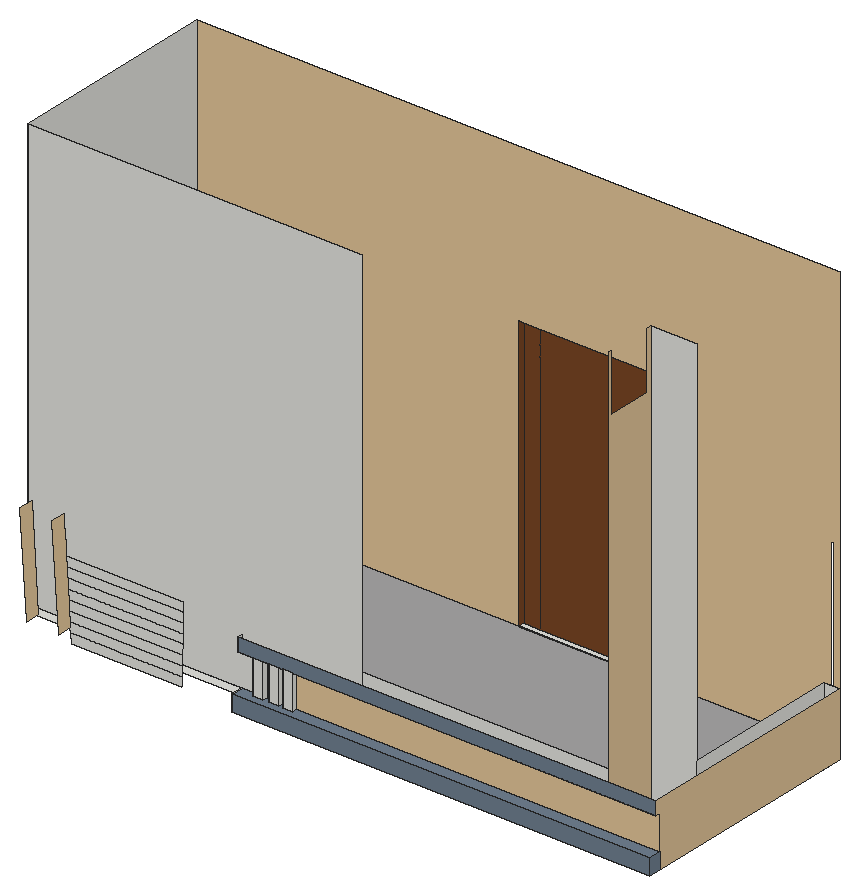
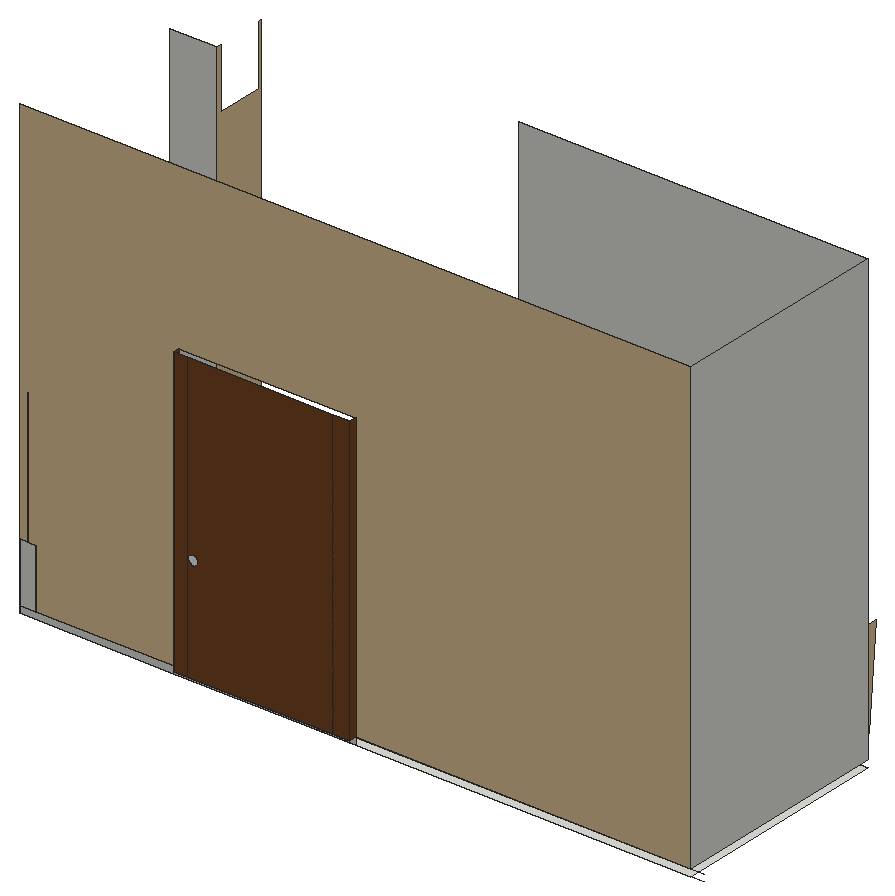
# SketchUp Ruby script. Lengths in inches.
U = 1.inch
M = Sketchup.active_model
def pt(a) = Geom::Point3d.new(a.map { |v| v * U })
def face(e, loops, mat)
  f = e.add_face(loops[0].map { |a| pt(a) })
  loops[1..].each { |l| e.add_face(l.map { |a| pt(a) }).erase! }
  f.material = f.back_material = mat if mat
  f
end
# faces: each face lists its corners as indices into pts; further lists are holes
def faces(e, pts, list, mat = nil) = list.each { |f| face(e, (f[0].is_a?(Array) ? f : [f]).map { |l| l.map { |i| pts[i] } }, mat) }
# xy, xz, yz: faces in a plane at the given z, y or x. An outline is a flat list of corners, or four numbers for a rectangle; further outlines are holes
def ring(l) = l.size == 4 ? [[l[0], l[1]], [l[2], l[1]], [l[2], l[3]], [l[0], l[3]]] : l.each_slice(2).to_a
def flat(e, list, mat, &to3) = list.each { |f| face(e, (f[0].is_a?(Array) ? f : [f]).map { |l| ring(l).map { |u, v| to3.(u, v) } }, mat) }
def xy(e, z, list, mat = nil) = flat(e, list, mat) { |x, y| [x, y, z] }
def xz(e, y, list, mat = nil) = flat(e, list, mat) { |x, z| [x, y, z] }
def yz(e, x, list, mat = nil) = flat(e, list, mat) { |y, z| [x, y, z] }
def lines(e, pts, list) = list.each { |a, b| e.add_line(pt(pts[a]), pt(pts[b])) }
# prism: a flat outline (further loops are holes) pulled along v
def prism(e, loops, v, mat = nil)
  f = face(e, loops, mat); d = Geom::Vector3d.new(v.map { |x| x * U })
  f.pushpull(f.normal.samedirection?(d) ? d.length : -d.length)
end
def box(e, o, s, mat = nil) = prism(e, [[o, [o[0] + s[0], o[1], o[2]], [o[0] + s[0], o[1] + s[1], o[2]], [o[0], o[1] + s[1], o[2]]]], [0, 0, s[2]], mat)
def at(x, y, z, deg = 0) = Geom::Transformation.translation(pt([x, y, z])) * Geom::Transformation.rotation(ORIGIN, Z_AXIS, deg.degrees)
def axes(o, x, y, z) = Geom::Transformation.new([*x, 0, *y, 0, *z, 0, *pt(o).to_a, 1])
def part(name) = M.definitions.add(name)
# library, detail: a bought-in or finely detailed component or shape, given as its bounding box
def library(name, o, s) = part(name).tap { |d| box(d.entities, o, s) }
def detail(e, o, s) = box(e.add_group.entities, o, s)
def put(e, d, t, mat = nil) = e.add_instance(d, t).tap { |i| i.material = mat if mat }
def group(e, t, mat = nil) = e.add_group.tap { |g| g.transformation = t; g.material = mat if mat }.entities
root = M.entities
M.materials.add("[0033_NavajoWhite]").color = [226, 197, 153]
M.materials.add("[0111_SlateGray]1").color = [112, 128, 144]
M.materials.add("[Stone Vein Gray]").color = [166, 165, 165]
M.materials.add("[Wood Cherry Original]").color = [152, 86, 42]
M.materials.add("[Wood Veneer 01]").color = [120, 70, 37]
xy(root,876,[[[676.39,210.26,773.27,472.7],[732.83,250.49,739.09,250.49,745.14,252.11,750.57,255.24,755,259.68,758.13,265.1,759.75,271.16,759.75,277.42,758.125,283.47,754.99,288.9,750.56,293.33,745.13,296.46,739.08,298.08,732.82,298.08,726.76,296.45,721.34,293.32,716.91,288.89,713.78,283.46,712.16,277.41,712.16,271.14,713.78,265.09,716.92,259.67,721.35,255.24,726.78,252.11],[729.45,399.49,735.72,399.49,741.77,401.11,747.19,404.24,751.625,408.68,754.75,414.1,756.375,420.16,756.375,426.42,754.75,432.47,751.62,437.9,747.19,442.33,741.76,445.46,735.71,447.08,729.44,447.08,723.39,445.45,717.96,442.32,713.54,437.89,710.4,432.46,708.78,426.41,708.79,420.14,710.41,414.09,713.54,408.67,717.97,404.24,723.4,401.11]],[773.27,210.26,926.08,472.7],[[926.08,210.26,1043.02,472.7],[965.39,250.49,971.66,250.49,977.71,252.11,983.13,255.24,987.5625,259.68,990.69,265.1,992.3125,271.16,992.3125,277.42,990.6875,283.47,987.55,288.9,983.12,293.33,977.7,296.46,971.64,298.08,965.38,298.08,959.33,296.45,953.9,293.32,949.47,288.89,946.34,283.46,944.72,277.41,944.72,271.14,946.35,265.09,949.48,259.67,953.91,255.24,959.34,252.11],[965.39,399.49,971.66,399.49,977.71,401.11,983.13,404.24,987.5625,408.68,990.69,414.1,992.3125,420.16,992.3125,426.42,990.6875,432.47,987.55,437.9,983.12,442.33,977.7,445.46,971.64,447.08,965.38,447.08,959.33,445.45,953.9,442.32,949.47,437.89,946.34,432.46,944.72,426.41,944.72,420.14,946.35,414.09,949.48,408.67,953.91,404.24,959.34,401.11]]],"[Wood Cherry Original]")
xy(root,882,[[732.83,250.49,726.78,252.11,721.35,255.24,716.92,259.67,713.78,265.09,712.16,271.14,712.16,277.41,713.78,283.46,716.91,288.89,721.34,293.32,726.76,296.45,732.82,298.08,739.08,298.08,745.13,296.46,750.56,293.33,754.99,288.9,758.125,283.47,759.75,277.42,759.75,271.16,758.13,265.1,755,259.68,750.57,255.24,745.14,252.11,739.09,250.49],[965.39,250.49,959.34,252.11,953.91,255.24,949.48,259.67,946.35,265.09,944.72,271.14,944.72,277.41,946.34,283.46,949.47,288.89,953.9,293.32,959.33,296.45,965.38,298.08,971.64,298.08,977.7,296.46,983.12,293.33,987.55,288.9,990.6875,283.47,992.3125,277.42,992.3125,271.16,990.69,265.1,987.5625,259.68,983.13,255.24,977.71,252.11,971.66,250.49],[729.45,399.49,723.4,401.11,717.97,404.24,713.54,408.67,710.41,414.09,708.79,420.14,708.78,426.41,710.4,432.46,713.54,437.89,717.96,442.32,723.39,445.45,729.44,447.08,735.71,447.08,741.76,445.46,747.19,442.33,751.62,437.9,754.75,432.47,756.375,426.42,756.375,420.16,754.75,414.1,751.625,408.68,747.19,404.24,741.77,401.11,735.72,399.49],[965.39,399.49,959.34,401.11,953.91,404.24,949.48,408.67,946.35,414.09,944.72,420.14,944.72,426.41,946.34,432.46,949.47,437.89,953.9,442.32,959.33,445.45,965.38,447.08,971.64,447.08,977.7,445.46,983.12,442.33,987.55,437.9,990.6875,432.47,992.3125,426.42,992.3125,420.16,990.69,414.1,987.5625,408.68,983.13,404.24,977.71,401.11,971.66,399.49]])
xy(root,888,[[[444,94.125,444,118.125,648,118.125,648,142.125,24,142.125,24,538.125,1224,538.125,1224,94.125],[676.39,210.26,1043.02,472.7],[1108.625,142.125,1118.15,142.125,1118.15,144.125,1184.28,144.125,1184.28,142.125,1193.3125,142.125,1193.3125,239.75,1108.625,239.75,1108.625,232.4375,1110.625,232.4375,1110.625,146.9375,1108.625,146.9375],[477.32,98.96,479.1,99.38,480.71,100.25,482.03,101.51,482.99,103.0625,483.52,104.8125,483.57,106.64,483.15,108.42,482.28,110.03,481.02,111.35,479.47,112.3125,477.72,112.84,475.89,112.89,474.11,112.47,472.5,111.6,471.18,110.34,470.22,108.79,469.69,107.04,469.64,105.21,470.0625,103.43,470.93,101.83,472.1875,100.5,473.74,99.54,475.49,99.01],[522.94,98.96,524.72,99.38,526.33,100.25,527.66,101.51,528.62,103.0625,529.14,104.8125,529.19,106.64,528.77,108.42,527.9,110.03,526.65,111.35,525.09,112.3125,523.34,112.84,521.52,112.89,519.74,112.47,518.13,111.6,516.8,110.34,515.84,108.79,515.32,107.04,515.27,105.21,515.6875,103.43,516.56,101.83,517.8125,100.5,519.37,99.54,521.12,99.01],[562.26,98.96,564.03,99.38,565.64,100.25,566.97,101.51,567.93,103.0625,568.45,104.8125,568.51,106.64,568.08,108.42,567.22,110.03,565.96,111.35,564.41,112.3125,562.65,112.84,560.83,112.89,559.05,112.47,557.44,111.6,556.11,110.34,555.15,108.79,554.63,107.04,554.58,105.21,555,103.43,555.87,101.83,557.125,100.5,558.68,99.54,560.43,99.01],[606.26,98.96,608.03,99.38,609.64,100.25,610.97,101.51,611.93,103.0625,612.45,104.8125,612.51,106.64,612.08,108.42,611.22,110.03,609.96,111.35,608.41,112.3125,606.65,112.84,604.83,112.89,603.05,112.47,601.44,111.6,600.11,110.34,599.15,108.79,598.63,107.04,598.58,105.21,599,103.43,599.87,101.83,601.125,100.5,602.68,99.54,604.43,99.01]]])
xy(root,891,[[477.32,98.96,475.49,99.01,473.74,99.54,472.1875,100.5,470.93,101.83,470.0625,103.43,469.64,105.21,469.69,107.04,470.22,108.79,471.18,110.34,472.5,111.6,474.11,112.47,475.89,112.89,477.72,112.84,479.47,112.3125,481.02,111.35,482.28,110.03,483.15,108.42,483.57,106.64,483.52,104.8125,482.99,103.0625,482.03,101.51,480.71,100.25,479.1,99.38],[522.94,98.96,521.12,99.01,519.37,99.54,517.8125,100.5,516.56,101.83,515.6875,103.43,515.27,105.21,515.32,107.04,515.84,108.79,516.8,110.34,518.13,111.6,519.74,112.47,521.52,112.89,523.34,112.84,525.09,112.3125,526.65,111.35,527.9,110.03,528.77,108.42,529.19,106.64,529.14,104.8125,528.62,103.0625,527.66,101.51,526.33,100.25,524.72,99.38],[562.26,98.96,560.43,99.01,558.68,99.54,557.125,100.5,555.87,101.83,555,103.43,554.58,105.21,554.63,107.04,555.15,108.79,556.11,110.34,557.44,111.6,559.05,112.47,560.83,112.89,562.65,112.84,564.41,112.3125,565.96,111.35,567.22,110.03,568.08,108.42,568.51,106.64,568.45,104.8125,567.93,103.0625,566.97,101.51,565.64,100.25,564.03,99.38],[606.26,98.96,604.43,99.01,602.68,99.54,601.125,100.5,599.87,101.83,599,103.43,598.58,105.21,598.63,107.04,599.15,108.79,600.11,110.34,601.44,111.6,603.05,112.47,604.83,112.89,606.65,112.84,608.41,112.3125,609.96,111.35,611.22,110.03,612.08,108.42,612.51,106.64,612.45,104.8125,611.93,103.0625,610.97,101.51,609.64,100.25,608.03,99.38]])
xy(root,900,[[624,538.125,939.8125,550.125]])
xy(root,900,[[24,142.125,1110.4375,142.125,1110.4375,239.75,1195.125,239.75,1195.125,538.125,24,538.125]],"[Stone Vein Gray]")
xy(root,918,[[444,94.125,1224,94.125,1224,118.125,545.1,118.125,545.1,109.125,526.42,109.125,526.42,118.125,519.47,118.125,519.47,109.125,500.8,109.125,500.8,118.125,490.66,118.125,490.66,109.125,471.99,109.125,471.99,118.125,444,118.125]],"[0111_SlateGray]1")
xy(root,982.5625,[[444,109.125,471.99,118.125],[490.66,109.125,500.8,118.125],[519.47,109.125,526.42,118.125]])
xy(root,982.5625,[[545.1,109.125,1224,118.125]],"[0111_SlateGray]1")
xz(root,94.125,[[444,888,1224,918]],"[0111_SlateGray]1")
xz(root,109.125,[[471.99,918,490.66,982.5625],[500.8,918,519.47,982.5625],[526.42,918,545.1,982.5625]])
xz(root,109.125,[[444,982.5625,1224,1006.5625]],"[0111_SlateGray]1")
xz(root,118.125,[[126.46,879.78,331.48,879.78,331.72,897.78,123.96,897.78],[123.96,897.78,331.72,897.78,331.96,915.78,122.1875,915.78,122.81,906.12],[122.1875,915.78,331.96,915.78,332.2,933.78,121.03,933.78],[490.66,918,500.8,982.5625],[519.47,918,526.42,982.5625],
  [121.03,933.78,332.2,933.78,332.45,951.78,119.86,951.78],[119.86,951.78,332.45,951.78,332.69,969.78,118.7,969.78],[118.7,969.78,332.69,969.78,332.93,987.78,117.54,987.78],[117.54,987.78,332.93,987.78,333.18,1005.78,116.38,1005.78],[116.38,1005.78,333.18,1005.78,333.42,1023.78,115.22,1023.78]])
xz(root,118.125,[[545.1,918,1224,982.5625]],"[0033_NavajoWhite]")
xz(root,142.125,[[24,900,648,1704],[648,900,1110.4375,1006.5625]])
xz(root,210.26,[[676.39,876,1043.02,888]],"[Wood Cherry Original]")
xz(root,239.75,[[1110.4375,900,1195.125,1704]])
xz(root,250.49,[[732.83,876,739.09,882],[965.39,876,971.66,882]])
xz(root,298.08,[[732.82,876,739.08,882],[965.38,876,971.64,882]])
xz(root,399.49,[[729.45,876,735.72,882],[965.39,876,971.66,882]])
xz(root,447.08,[[729.44,876,735.71,882],[965.38,876,971.64,882]])
xz(root,472.7,[[676.39,876,1043.02,888]],"[Wood Cherry Original]")
xz(root,538.125,[[624,888,939.8125,900],[939.8125,888,1224,900],[1195.125,900,1224,1006.5625]])
xz(root,538.125,[[24,900,624,900,624,1411.875,939.8125,1411.875,939.8125,900,1195.125,900,1195.125,1006.5625,1208.3,1006.5625,1208.3,1246.5625,1212.3,1246.5625,1212.3,1006.5625,1224,1006.5625,1224,1704,24,1704]],"[0033_NavajoWhite]")
xz(root,550.125,[[624,900,654,1411.875],[[654,900,915.8125,1411.875],[904.46,1081.11,902.13,1081.41,899.96,1082.3125,898.09,1083.74,896.66,1085.61,895.77,1087.78,895.46,1090.11,895.77,1092.44,896.66,1094.61,898.09,1096.47,899.96,1097.9,902.13,1098.8,904.46,1099.11,906.79,1098.8,908.96,1097.9,910.82,1096.47,912.25,1094.61,913.15,1092.44,913.46,1090.11,913.15,1087.78,912.25,1085.61,910.82,1083.74,908.96,1082.3125,906.79,1081.41]],[915.8125,900,939.8125,1411.875]],"[Wood Veneer 01]")
yz(root,24,[[142.125,900,538.125,1704]])
yz(root,444,[[94.125,888,118.125,918],[109.125,982.5625,118.125,1006.5625]])
yz(root,471.99,[[109.125,918,118.125,982.5625]])
yz(root,490.66,[[109.125,918,118.125,982.5625]])
yz(root,500.8,[[109.125,918,118.125,982.5625]])
yz(root,519.47,[[109.125,918,118.125,982.5625]])
yz(root,526.42,[[109.125,918,118.125,982.5625]])
yz(root,545.1,[[109.125,918,118.125,982.5625]])
yz(root,624,[[538.125,900,550.125,1411.875]],"[Wood Veneer 01]")
yz(root,676.39,[[210.26,876,472.7,888]])
yz(root,712.16,[[271.14,876,277.41,882]])
yz(root,756.375,[[420.16,876,426.42,882]])
yz(root,759.75,[[271.16,876,277.42,882]])
yz(root,939.8125,[[538.125,900,550.125,1411.875]],"[Wood Veneer 01]")
yz(root,944.72,[[271.14,876,277.41,882],[420.14,876,426.41,882]])
yz(root,992.3125,[[271.16,876,277.42,882],[420.16,876,426.42,882]])
yz(root,1043.02,[[210.26,876,472.7,888]],"[Wood Cherry Original]")
yz(root,1110.4375,[[142.125,900,142.125,1704,146.89,1704,146.89,1596.63,229.71,1596.63,229.71,1704,239.75,1704,239.75,900]],"[0033_NavajoWhite]")
yz(root,1195.125,[[239.75,900,538.125,1006.5625]])
yz(root,1224,[[118.125,888,538.125,888,538.125,1006.5625,109.125,1006.5625,109.125,982.5625,118.125,982.5625]],"[0033_NavajoWhite]")
yz(root,1224,[[94.125,888,118.125,918]],"[0111_SlateGray]1")
p = [[732.83,250.49,876],[726.78,252.11,876],[726.78,252.11,882],[732.83,250.49,882],[745.14,252.11,876],[739.09,250.49,876],
  [739.09,250.49,882],[745.14,252.11,882],[965.39,250.49,876],[959.34,252.11,876],[959.34,252.11,882],[965.39,250.49,882],
  [977.71,252.11,876],[971.66,250.49,876],[971.66,250.49,882],[977.71,252.11,882],[721.35,255.24,876],[721.35,255.24,882],
  [750.57,255.24,876],[750.57,255.24,882],[953.91,255.24,876],[953.91,255.24,882],[983.13,255.24,876],[983.13,255.24,882],
  [716.92,259.67,876],[716.92,259.67,882],[755,259.68,876],[755,259.68,882],[949.48,259.67,876],[949.48,259.67,882],
  [987.5625,259.68,876],[987.5625,259.68,882],[713.78,265.09,876],[713.78,265.09,882],[758.13,265.1,876],[758.13,265.1,882],
  [946.35,265.09,876],[946.35,265.09,882],[990.69,265.1,876],[990.69,265.1,882],[712.16,271.14,876],[712.16,271.14,882],
  [759.75,271.16,876],[759.75,271.16,882],[944.72,271.14,876],[944.72,271.14,882],[992.3125,271.16,876],[992.3125,271.16,882],
  [712.16,277.41,876],[713.78,283.46,876],[713.78,283.46,882],[712.16,277.41,882],[758.125,283.47,876],[759.75,277.42,876],
  [759.75,277.42,882],[758.125,283.47,882],[944.72,277.41,876],[946.34,283.46,876],[946.34,283.46,882],[944.72,277.41,882],
  [990.6875,283.47,876],[992.3125,277.42,876],[992.3125,277.42,882],[990.6875,283.47,882],[716.91,288.89,876],[716.91,288.89,882],
  [754.99,288.9,876],[754.99,288.9,882],[949.47,288.89,876],[949.47,288.89,882],[987.55,288.9,876],[987.55,288.9,882],
  [721.34,293.32,876],[721.34,293.32,882],[750.56,293.33,876],[750.56,293.33,882],[953.9,293.32,876],[953.9,293.32,882],
  [983.12,293.33,876],[983.12,293.33,882],[726.76,296.45,876],[726.76,296.45,882],[745.13,296.46,876],[745.13,296.46,882],
  [959.33,296.45,876],[959.33,296.45,882],[977.7,296.46,876],[977.7,296.46,882],[732.82,298.08,876],[732.82,298.08,882],
  [739.08,298.08,876],[739.08,298.08,882],[965.38,298.08,876],[965.38,298.08,882],[971.64,298.08,876],[971.64,298.08,882],
  [729.45,399.49,876],[723.4,401.11,876],[723.4,401.11,882],[729.45,399.49,882],[741.77,401.11,876],[735.72,399.49,876],
  [735.72,399.49,882],[741.77,401.11,882],[965.39,399.49,876],[959.34,401.11,876],[959.34,401.11,882],[965.39,399.49,882],
  [977.71,401.11,876],[971.66,399.49,876],[971.66,399.49,882],[977.71,401.11,882],[717.97,404.24,876],[717.97,404.24,882],
  [747.19,404.24,876],[747.19,404.24,882],[953.91,404.24,876],[953.91,404.24,882],[983.13,404.24,876],[983.13,404.24,882],
  [713.54,408.67,876],[713.54,408.67,882],[751.625,408.68,876],[751.625,408.68,882],[949.48,408.67,876],[949.48,408.67,882],
  [987.5625,408.68,876],[987.5625,408.68,882],[710.41,414.09,876],[710.41,414.09,882],[754.75,414.1,876],[754.75,414.1,882],
  [946.35,414.09,876],[946.35,414.09,882],[990.69,414.1,876],[990.69,414.1,882],[708.79,420.14,876],[708.79,420.14,882],
  [756.375,420.16,876],[756.375,420.16,882],[944.72,420.14,876],[944.72,420.14,882],[992.3125,420.16,876],[992.3125,420.16,882],
  [708.78,426.41,876],[708.78,426.41,882],[710.4,432.46,876],[710.4,432.46,882],[754.75,432.47,876],[756.375,426.42,876],
  [756.375,426.42,882],[754.75,432.47,882],[944.72,426.41,876],[946.34,432.46,876],[946.34,432.46,882],[944.72,426.41,882],
  [990.6875,432.47,876],[992.3125,426.42,876],[992.3125,426.42,882],[990.6875,432.47,882],[713.54,437.89,876],[713.54,437.89,882],
  [751.62,437.9,876],[751.62,437.9,882],[949.47,437.89,876],[949.47,437.89,882],[987.55,437.9,876],[987.55,437.9,882],
  [717.96,442.32,876],[717.96,442.32,882],[747.19,442.33,876],[747.19,442.33,882],[953.9,442.32,876],[953.9,442.32,882],
  [983.12,442.33,876],[983.12,442.33,882],[723.39,445.45,876],[723.39,445.45,882],[741.76,445.46,876],[741.76,445.46,882],
  [959.33,445.45,876],[959.33,445.45,882],[977.7,445.46,876],[977.7,445.46,882],[729.44,447.08,876],[729.44,447.08,882],
  [735.71,447.08,876],[735.71,447.08,882],[965.38,447.08,876],[965.38,447.08,882],[971.64,447.08,876],[971.64,447.08,882],
  [475.49,99.01,888],[473.74,99.54,888],[473.74,99.54,891],[475.49,99.01,891],[477.32,98.96,888],[477.32,98.96,891],
  [479.1,99.38,888],[479.1,99.38,891],[521.12,99.01,888],[519.37,99.54,888],[519.37,99.54,891],[521.12,99.01,891],
  [522.94,98.96,888],[522.94,98.96,891],[524.72,99.38,888],[524.72,99.38,891],[560.43,99.01,888],[558.68,99.54,888],
  [558.68,99.54,891],[560.43,99.01,891],[562.26,98.96,888],[562.26,98.96,891],[564.03,99.38,888],[564.03,99.38,891],
  [604.43,99.01,888],[602.68,99.54,888],[602.68,99.54,891],[604.43,99.01,891],[606.26,98.96,888],[606.26,98.96,891],
  [608.03,99.38,888],[608.03,99.38,891],[480.71,100.25,888],[480.71,100.25,891],[526.33,100.25,888],[526.33,100.25,891],
  [565.64,100.25,888],[565.64,100.25,891],[609.64,100.25,888],[609.64,100.25,891],[472.1875,100.5,888],[472.1875,100.5,891],
  [517.8125,100.5,888],[517.8125,100.5,891],[557.125,100.5,888],[557.125,100.5,891],[601.125,100.5,888],[601.125,100.5,891],
  [482.03,101.51,888],[482.03,101.51,891],[527.66,101.51,888],[527.66,101.51,891],[566.97,101.51,888],[566.97,101.51,891],
  [610.97,101.51,888],[610.97,101.51,891],[470.93,101.83,888],[470.93,101.83,891],[516.56,101.83,888],[516.56,101.83,891],
  [555.87,101.83,888],[555.87,101.83,891],[599.87,101.83,888],[599.87,101.83,891],[482.99,103.0625,888],[482.99,103.0625,891],
  [528.62,103.0625,888],[528.62,103.0625,891],[567.93,103.0625,888],[567.93,103.0625,891],[611.93,103.0625,888],[611.93,103.0625,891],
  [470.0625,103.43,888],[470.0625,103.43,891],[515.6875,103.43,888],[515.6875,103.43,891],[555,103.43,888],[555,103.43,891],
  [599,103.43,888],[599,103.43,891],[483.52,104.8125,888],[483.52,104.8125,891],[529.14,104.8125,888],[529.14,104.8125,891],
  [568.45,104.8125,888],[568.45,104.8125,891],[612.45,104.8125,888],[612.45,104.8125,891],[469.64,105.21,888],[469.64,105.21,891],
  [515.27,105.21,888],[515.27,105.21,891],[554.58,105.21,888],[554.58,105.21,891],[598.58,105.21,888],[598.58,105.21,891],
  [483.57,106.64,888],[483.57,106.64,891],[529.19,106.64,888],[529.19,106.64,891],[568.51,106.64,888],[568.51,106.64,891],
  [612.51,106.64,888],[612.51,106.64,891],[469.69,107.04,888],[469.69,107.04,891],[515.32,107.04,888],[515.32,107.04,891],
  [554.63,107.04,888],[554.63,107.04,891],[598.63,107.04,888],[598.63,107.04,891],[483.15,108.42,888],[483.15,108.42,891],
  [528.77,108.42,888],[528.77,108.42,891],[568.08,108.42,888],[568.08,108.42,891],[612.08,108.42,888],[612.08,108.42,891],
  [470.22,108.79,888],[470.22,108.79,891],[515.84,108.79,888],[515.84,108.79,891],[555.15,108.79,888],[555.15,108.79,891],
  [599.15,108.79,888],[599.15,108.79,891],[482.28,110.03,888],[482.28,110.03,891],[527.9,110.03,888],[527.9,110.03,891],
  [567.22,110.03,888],[567.22,110.03,891],[611.22,110.03,888],[611.22,110.03,891],[471.18,110.34,888],[471.18,110.34,891],
  [516.8,110.34,888],[516.8,110.34,891],[556.11,110.34,888],[556.11,110.34,891],[600.11,110.34,888],[600.11,110.34,891],
  [481.02,111.35,888],[481.02,111.35,891],[526.65,111.35,888],[526.65,111.35,891],[565.96,111.35,888],[565.96,111.35,891],
  [609.96,111.35,888],[609.96,111.35,891],[472.5,111.6,888],[472.5,111.6,891],[518.13,111.6,888],[518.13,111.6,891],
  [557.44,111.6,888],[557.44,111.6,891],[601.44,111.6,888],[601.44,111.6,891],[479.47,112.3125,888],[479.47,112.3125,891],
  [525.09,112.3125,888],[525.09,112.3125,891],[564.41,112.3125,888],[564.41,112.3125,891],[608.41,112.3125,888],[608.41,112.3125,891],
  [474.11,112.47,888],[474.11,112.47,891],[519.74,112.47,888],[519.74,112.47,891],[559.05,112.47,888],[559.05,112.47,891],
  [603.05,112.47,888],[603.05,112.47,891],[477.72,112.84,888],[477.72,112.84,891],[523.34,112.84,888],[523.34,112.84,891],
  [562.65,112.84,888],[562.65,112.84,891],[606.65,112.84,888],[606.65,112.84,891],[475.89,112.89,888],[475.89,112.89,891],
  [521.52,112.89,888],[521.52,112.89,891],[560.83,112.89,888],[560.83,112.89,891],[604.83,112.89,888],[604.83,112.89,891],
  [50.76,118.125,1093.03],[62.81,118.125,906.12],[62.81,91.125,906.12],[50.76,91.125,1093.03],[111.74,118.125,1077.78],[110.76,118.125,1093.03],
  [110.76,91.125,1093.03],[122.81,91.125,906.12],[122.81,118.125,906.12],[122.1875,118.125,915.78],[121.03,118.125,933.78],[119.86,118.125,951.78],
  [118.7,118.125,969.78],[117.54,118.125,987.78],[116.38,118.125,1005.78],[115.22,118.125,1023.78],[114.0625,118.125,1041.78],[112.9,118.125,1059.78],
  [24,538.125,900],[0,538.125,900],[24,538.125,888],[0,538.125,888]]
faces(root,p,[[0,1,2,3],[4,5,6,7],[8,9,10,11],[12,13,14,15],[1,16,17,2],[18,4,7,19],[9,20,21,10],[22,12,15,23],
  [16,24,25,17],[26,18,19,27],[20,28,29,21],[30,22,23,31],[24,32,33,25],[34,26,27,35],[28,36,37,29],[38,30,31,39],
  [32,40,41,33],[42,34,35,43],[36,44,45,37],[46,38,39,47],[48,49,50,51],[52,53,54,55],[56,57,58,59],[60,61,62,63],
  [49,64,65,50],[66,52,55,67],[57,68,69,58],[70,60,63,71],[64,72,73,65],[74,66,67,75],[68,76,77,69],[78,70,71,79],
  [72,80,81,73],[82,74,75,83],[76,84,85,77],[86,78,79,87],[80,88,89,81],[90,82,83,91],[84,92,93,85],[94,86,87,95],
  [96,97,98,99],[100,101,102,103],[104,105,106,107],[108,109,110,111],[97,112,113,98],[114,100,103,115],[105,116,117,106],[118,108,111,119],
  [112,120,121,113],[122,114,115,123],[116,124,125,117],[126,118,119,127],[120,128,129,121],[130,122,123,131],[124,132,133,125],[134,126,127,135],
  [128,136,137,129],[138,130,131,139],[132,140,141,133],[142,134,135,143],[136,144,145,137],[144,146,147,145],[148,149,150,151],[152,153,154,155],
  [156,157,158,159],[146,160,161,147],[162,148,151,163],[153,164,165,154],[166,156,159,167],[160,168,169,161],[170,162,163,171],[164,172,173,165],
  [174,166,167,175],[168,176,177,169],[178,170,171,179],[172,180,181,173],[182,174,175,183],[176,184,185,177],[186,178,179,187],[180,188,189,181],
  [190,182,183,191],[192,193,194,195],[196,192,195,197],[198,196,197,199],[200,201,202,203],[204,200,203,205],[206,204,205,207],[208,209,210,211],
  [212,208,211,213],[214,212,213,215],[216,217,218,219],[220,216,219,221],[222,220,221,223],[224,198,199,225],[226,206,207,227],[228,214,215,229],
  [230,222,223,231],[193,232,233,194],[201,234,235,202],[209,236,237,210],[217,238,239,218],[240,224,225,241],[242,226,227,243],[244,228,229,245],
  [246,230,231,247],[232,248,249,233],[234,250,251,235],[236,252,253,237],[238,254,255,239],[256,240,241,257],[258,242,243,259],[260,244,245,261],
  [262,246,247,263],[248,264,265,249],[250,266,267,251],[252,268,269,253],[254,270,271,255],[272,256,257,273],[274,258,259,275],[276,260,261,277],
  [278,262,263,279],[264,280,281,265],[266,282,283,267],[268,284,285,269],[270,286,287,271],[288,272,273,289],[290,274,275,291],[292,276,277,293],
  [294,278,279,295],[280,296,297,281],[282,298,299,283],[284,300,301,285],[286,302,303,287],[304,288,289,305],[306,290,291,307],[308,292,293,309],
  [310,294,295,311],[296,312,313,297],[298,314,315,299],[300,316,317,301],[302,318,319,303],[320,304,305,321],[322,306,307,323],[324,308,309,325],
  [326,310,311,327],[312,328,329,313],[314,330,331,315],[316,332,333,317],[318,334,335,319],[336,320,321,337],[338,322,323,339],[340,324,325,341],
  [342,326,327,343],[328,344,345,329],[330,346,347,331],[332,348,349,333],[334,350,351,335],[352,336,337,353],[354,338,339,355],[356,340,341,357],
  [358,342,343,359],[344,360,361,345],[346,362,363,347],[348,364,365,349],[350,366,367,351],[368,352,353,369],[370,354,355,371],[372,356,357,373],
  [374,358,359,375],[360,376,377,361],[362,378,379,363],[364,380,381,365],[366,382,383,367],[376,368,369,377],[378,370,371,379],[380,372,373,381],
  [382,374,375,383]])
faces(root,p,[[384,385,386,387],[388,389,390,391,392,393,394,395,396,397,398,399,400,401]],"[0033_NavajoWhite]")
lines(root,p,[[402,403],[404,405]])
